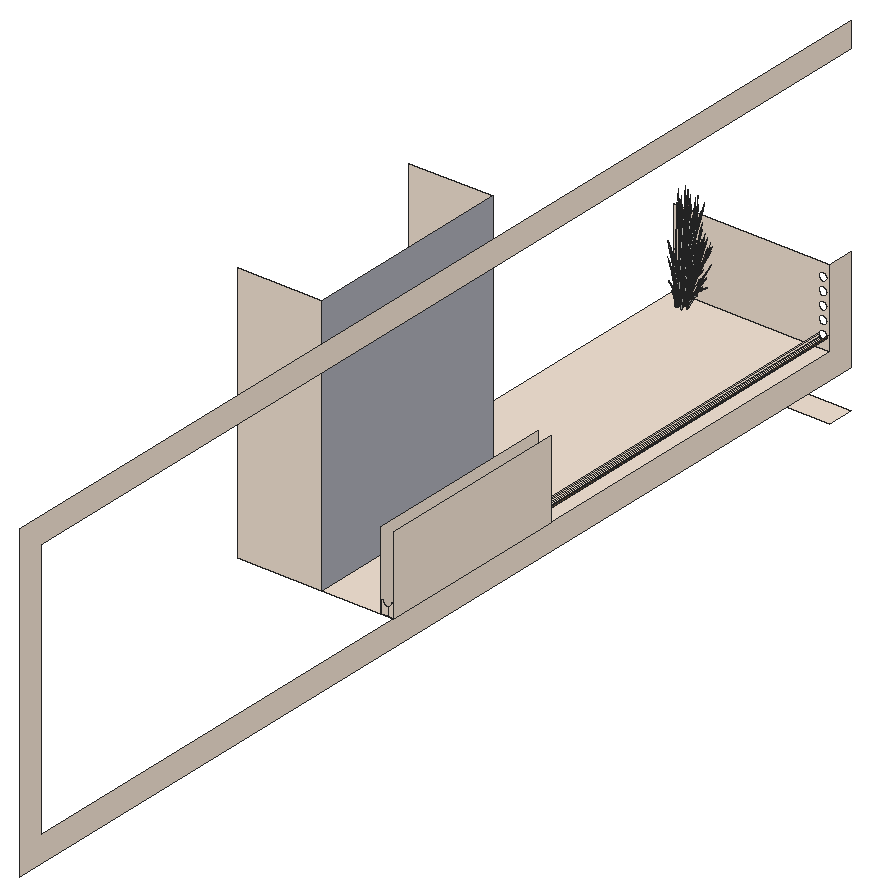
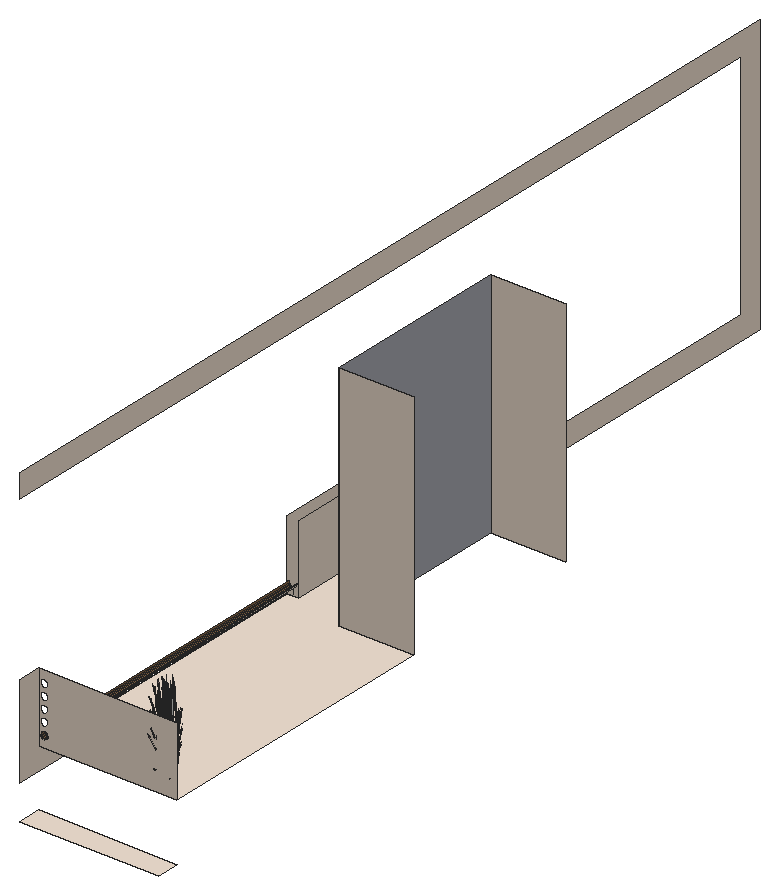
# SketchUp Ruby script. Lengths in inches.
U = 1.inch
M = Sketchup.active_model
def pt(a) = Geom::Point3d.new(a.map { |v| v * U })
def face(e, loops, mat)
  f = e.add_face(loops[0].map { |a| pt(a) })
  loops[1..].each { |l| e.add_face(l.map { |a| pt(a) }).erase! }
  f.material = f.back_material = mat if mat
  f
end
# faces: each face lists its corners as indices into pts; further lists are holes
def faces(e, pts, list, mat = nil) = list.each { |f| face(e, (f[0].is_a?(Array) ? f : [f]).map { |l| l.map { |i| pts[i] } }, mat) }
# xy, xz, yz: faces in a plane at the given z, y or x. An outline is a flat list of corners, or four numbers for a rectangle; further outlines are holes
def ring(l) = l.size == 4 ? [[l[0], l[1]], [l[2], l[1]], [l[2], l[3]], [l[0], l[3]]] : l.each_slice(2).to_a
def flat(e, list, mat, &to3) = list.each { |f| face(e, (f[0].is_a?(Array) ? f : [f]).map { |l| ring(l).map { |u, v| to3.(u, v) } }, mat) }
def xy(e, z, list, mat = nil) = flat(e, list, mat) { |x, y| [x, y, z] }
def xz(e, y, list, mat = nil) = flat(e, list, mat) { |x, z| [x, y, z] }
def yz(e, x, list, mat = nil) = flat(e, list, mat) { |y, z| [x, y, z] }
def lines(e, pts, list) = list.each { |a, b| e.add_line(pt(pts[a]), pt(pts[b])) }
# prism: a flat outline (further loops are holes) pulled along v
def prism(e, loops, v, mat = nil)
  f = face(e, loops, mat); d = Geom::Vector3d.new(v.map { |x| x * U })
  f.pushpull(f.normal.samedirection?(d) ? d.length : -d.length)
end
def box(e, o, s, mat = nil) = prism(e, [[o, [o[0] + s[0], o[1], o[2]], [o[0] + s[0], o[1] + s[1], o[2]], [o[0], o[1] + s[1], o[2]]]], [0, 0, s[2]], mat)
def at(x, y, z, deg = 0) = Geom::Transformation.translation(pt([x, y, z])) * Geom::Transformation.rotation(ORIGIN, Z_AXIS, deg.degrees)
def axes(o, x, y, z) = Geom::Transformation.new([*x, 0, *y, 0, *z, 0, *pt(o).to_a, 1])
def part(name) = M.definitions.add(name)
# library, detail: a bought-in or finely detailed component or shape, given as its bounding box
def library(name, o, s) = part(name).tap { |d| box(d.entities, o, s) }
def detail(e, o, s) = box(e.add_group.entities, o, s)
def put(e, d, t, mat = nil) = e.add_instance(d, t).tap { |i| i.material = mat if mat }
def group(e, t, mat = nil) = e.add_group.tap { |g| g.transformation = t; g.material = mat if mat }.entities
root = M.entities
M.materials.add("C01_Vanilla_Cream").color = [244, 228, 212]
M.materials.add("LightPink_Translucent").color = [144, 107, 117]
M.materials["LightPink_Translucent"].alpha = 0.75
M.materials.add("Marble_20_1K").color = [172, 173, 182]
M.materials.add("Wood_Floor_01_1K").color = [146, 111, 76]
c1 = part("blade")
p = [[2.15,0.21,22],[0,0.17,0],[0.09,0.45,0],[2.18,0.31,22],[2.29,0.31,22],[0.38,0.45,0],
  [2.48,0.24,33],[2.49,0.24,33],[2.48,0.22,33]]
faces(c1.entities,p,[[0,1,2,3],[4,5,2,3],[6,3,4,7],[8,0,3,6]])
c2 = part("seeds")
p = [[0.3,-0.1,1.38],[-0.01,-0.03,1.59],[-0.01,-0.03,0.03],[0.14,-0.07,-0.07],[0.29,-0.03,3],[0.15,0.01,3.11]]
faces(c2.entities,p,[[0,1,2,3],[1,0,4,5]],"LightPink_Translucent")
c3 = part("blade with seeds")
put(c3.entities,c1,at(0,0,0))
put(c3.entities,c2,axes([2.4,0.25,30.99],[1.5799,-0.05474,1.17369],[-0.12525,1.92788,0.29478],[-0.07173,-0.02425,1.56792]))
xy(root,132,[[288,468,360,480]],"C01_Vanilla_Cream")
xy(root,162,[[326.85,216,354,216,354,306.76,360,306.76,360,468,288,468,288,314.71,326.85,314.71],[354,216,360,306.76]],"C01_Vanilla_Cream")
xz(root,216,[[288,162,326.85,282],[354,162,357,162,357,166,356.48,166.07,356,166.27,355.59,166.59,355.27,167,355.07,167.48,355,168,354,168],[357,162,360,162,360,168,359,168,358.93,167.48,358.73,167,358.41,166.59,358,166.27,357.52,166.07,357,166]],"C01_Vanilla_Cream")
xz(root,306.76,[[354,162,354,168,355,168,355.07,167.48,355.27,167,355.59,166.59,356,166.27,356.48,166.07,357,166,357,162],[357,162,357,166,357.52,166.07,358,166.27,358.41,166.59,358.73,167,358.93,167.48,359,168,360,168,360,162]],"C01_Vanilla_Cream")
xz(root,314.71,[[288,162,326.85,282]],"C01_Vanilla_Cream")
xz(root,468,[[[288,162,360,198],[357,190,356.48,190.07,356,190.27,355.59,190.59,355.27,191,355.07,191.48,355,192,355.07,192.52,355.27,193,355.59,193.41,356,193.73,356.48,193.93,357,194,357.52,193.93,358,193.73,358.41,193.41,358.73,193,358.93,192.52,359,192,358.93,191.48,358.73,191,358.41,190.59,358,190.27,357.52,190.07],[357,184,356.48,184.07,356,184.27,355.59,184.59,355.27,185,355.07,185.48,355,186,355.07,186.52,355.27,187,355.59,187.41,356,187.73,356.48,187.93,357,188,357.52,187.93,358,187.73,358.41,187.41,358.73,187,358.93,186.52,359,186,358.93,185.48,358.73,185,358.41,184.59,358,184.27,357.52,184.07],[357,178,356.48,178.07,356,178.27,355.59,178.59,355.27,179,355.07,179.48,355,180,355.07,180.52,355.27,181,355.59,181.41,356,181.73,356.48,181.93,357,182,357.52,181.93,358,181.73,358.41,181.41,358.73,181,358.93,180.52,359,180,358.93,179.48,358.73,179,358.41,178.59,358,178.27,357.52,178.07],[357,172,356.48,172.07,356,172.27,355.59,172.59,355.27,173,355.07,173.48,355,174,355.07,174.52,355.27,175,355.59,175.41,356,175.73,356.48,175.93,357,176,357.52,175.93,358,175.73,358.41,175.41,358.73,175,358.93,174.52,359,174,358.93,173.48,358.73,173,358.41,172.59,358,172.27,357.52,172.07],[357,166,356.48,166.07,356,166.27,355.59,166.59,355.27,167,355.07,167.48,355,168,355.07,168.52,355.27,169,355.59,169.41,356,169.73,356.48,169.93,357,170,357.52,169.93,358,169.73,358.41,169.41,358.73,169,358.93,168.52,359,168,358.93,167.48,358.73,167,358.41,166.59,358,166.27,357.52,166.07]]],"C01_Vanilla_Cream")
yz(root,326.85,[[216,162,314.71,282]],"Marble_20_1K")
yz(root,354,[[216,162,306.76,198]],"C01_Vanilla_Cream")
yz(root,360,[[0,150,480,150,480,198,468,198,468,162,12,162,12,282,480,282,480,294,0,294],[216,162,306.76,198]],"C01_Vanilla_Cream")
p = [[357,306.76,166],[356.48,306.76,166.07],[356.48,468,166.07],[357,468,166],[357.52,306.76,166.07],[357.52,468,166.07],
  [356,306.76,166.27],[356,468,166.27],[358,306.76,166.27],[358,468,166.27],[355.59,306.76,166.59],[355.59,468,166.59],
  [358.41,306.76,166.59],[358.41,468,166.59],[355.27,306.76,167],[355.27,468,167],[358.73,306.76,167],[358.73,468,167],
  [355.07,306.76,167.48],[355.07,468,167.48],[358.93,306.76,167.48],[358.93,468,167.48],[355,306.76,168],[355,468,168],
  [359,306.76,168],[359,468,168]]
faces(root,p,[[0,1,2,3],[1,6,7,2],[6,10,11,7],[10,14,15,11],[14,18,19,15],[18,22,23,19]],"C01_Vanilla_Cream")
faces(root,p,[[4,0,3,5],[8,4,5,9],[12,8,9,13],[16,12,13,17],[20,16,17,21],[24,20,21,25]],"Wood_Floor_01_1K")
put(root,c3,axes([297.36,461.41,163.12],[0.0901,-0.02681,1.32257],[0.54199,0.14755,-0.20205],[0.01585,0.1663,0.22528]))
put(root,c3,axes([297.48,461.5625,165.39],[-0.16784,0.37886,-0.2656],[-0.48968,-0.1105,0.3429],[0.0449,0.15254,0.65611]))
put(root,c3,axes([298.75,459.68,163.66],[-0.27012,0.44393,-0.33554],[-0.56127,-0.21365,0.16149],[0,0.10233,1.07733]))
put(root,c3,axes([298.47,457.17,165.55],[0.41024,-0.16744,0.04823],[0.2008,0.30532,0.37966],[-0.03962,-0.13459,0.57892]))
put(root,c3,axes([297.13,462.23,165.54],[0.07057,0.07933,1.31208],[0.56952,0.03117,-0.2075],[0.05727,0.17496,0.10523]))
put(root,c3,axes([299.82,459.41,163.86],[-0.43742,-0.35886,0.13232],[0.44081,-0.34807,0.26315],[-0.04831,0.07329,1.20305]))
put(root,c3,axes([298.3125,459.2,163.65],[0,-0.57005,0],[0.69617,0,0],[0,0,1.34592]))
put(root,c3,axes([298.32,457.2,165.55],[0.54859,0.1288,0.36002],[-0.18759,0.42344,0.29685],[-0.03297,-0.16652,0.74497]))
put(root,c3,axes([297.66,459.31,163.82],[0.6273,0.23878,0.18048],[-0.3019,0.49615,0.37502],[0,-0.11437,1.20407]))
put(root,c3,axes([298.66,459.43,163.72],[0,0.56976,-0.04228],[-0.69617,0,0],[0,0.01791,1.34526]))
put(root,c3,axes([297.46,458.97,164.04],[-0.60457,0.03041,0.33554],[-0.05467,-0.50484,-0.16149],[0.10823,-0.05117,1.07733]))
put(root,c3,axes([297.43,461.16,165.79],[0.16784,-0.37886,0.2656],[0.48968,0.1105,-0.3429],[0.0449,0.15254,0.65611]))
put(root,c3,axes([297.18,458.11,163.86],[-0.16083,0.48962,0.13232],[-0.58854,-0.13856,0.26315],[0.10167,-0.00238,1.20305]))
put(root,c3,axes([298.33,460.53,163.72],[0.24206,0.56598,-0.04509],[-0.69162,0.19832,0],[0.00845,0.01976,1.2913]))
put(root,c3,axes([296.89,457.5,163.78],[-0.34808,-0.49367,0],[0.58235,-0.27531,-0.38706],[0.13264,-0.0627,1.22783]))
put(root,c3,axes([297.53,461.22,165.74],[0.26572,0.40059,-0.53284],[-0.54698,0.22325,0.0643],[0.06214,0.19355,0.75375]))
put(root,c3,axes([300.33,459.79,163.65],[-0.69582,-0.00394,-0.03732],[0,-0.55062,0.37457],[-0.02187,0.12535,1.18764]))
put(root,c3,axes([298.96,458.13,163.86],[-0.59825,0.13076,0.13232],[-0.14773,-0.48663,0.26315],[0.05336,0.0709,1.20305]))
put(root,c3,axes([298.35,456.31,164.07],[0.07142,0.28728,0.86145],[-0.3962,-0.15911,0.63294],[0.04263,-0.1471,0.18974]))
put(root,c3,axes([298.09,462.52,166.23],[0.38473,-0.28263,-0.04866],[0.35252,0.30954,-0.22062],[0.02482,0.08771,0.72768]))
put(root,c3,axes([297.98,458.84,163.77],[-0.46162,0.4471,0.34316],[-0.54842,-0.39467,0.13466],[0.11129,-0.04462,1.19142]))
put(root,c3,axes([298.77,459.55,163.66],[0.38863,0.31822,0],[-0.38863,0.31822,0],[0,0,1.2695]))
put(root,c3,axes([298.77,459.18,164.04],[0.27012,-0.44393,0.33554],[0.56127,0.21365,-0.16149],[0,0.10233,1.07733]))
put(root,c3,axes([298.53,460.72,163.65],[0.56127,0.22118,0],[-0.27012,0.45959,0],[0,0,1.31215]))
put(root,c3,axes([297.73,461.3,165.51],[0.54728,0.1235,-0.38324],[-0.18759,0.42344,-0.29685],[0.05018,0.17048,0.7333]))
put(root,c3,axes([297.26,461.32,165.78],[0.54481,-0.22937,-0.0912],[0.26773,0.4071,-0.50621],[0.07188,0.17155,0.76918]))
put(root,c3,axes([298.58,459.07,163.79],[-0.70367,-0.1038,0.36899],[0.1432,-0.58624,0.1448],[0.10283,0.05661,1.2811]))
put(root,c3,axes([300.05,456.78,165.53],[-0.05654,0.03763,1.33037],[-0.55396,-0.12696,-0.12571],[-0.02005,-0.16422,0.23543]))
put(root,c3,axes([299.61,457.86,165.78],[-0.61188,-0.02441,-0.0912],[0.01672,-0.46217,-0.50621],[0.0425,-0.178,0.76918]))
put(root,c3,axes([300.18,459.87,163.52],[-0.38863,0.30738,-0.23233],[-0.38863,-0.30738,0.23233],[0,0.09901,1.0423]))
put(root,c3,axes([299.07,459.8125,163.57],[0.20414,0.45107,-0.51909],[-0.58805,0.16245,-0.13624],[0.02256,0.15274,1.1458]))
put(root,c3,axes([298.78,459.33,163.65],[0.62289,0,0],[0,0.51004,0],[0,0,1.33805]))
put(root,c3,axes([299.37,457.94,165.79],[-0.3767,0.25939,0.2656],[-0.3566,-0.29618,-0.3429],[0.05426,-0.15048,0.65611]))
put(root,c3,axes([298.19,458.77,164.04],[-0.33445,-0.41351,0.33554],[0.50659,-0.29119,-0.16149],[0.10823,0.05117,1.07733]))
put(root,c3,axes([297.58,458.87,164],[-0.06488,-0.56215,-0.21822],[0.6757,-0.03399,-0.37502],[0.11898,-0.07488,1.19781]))
put(root,c3,axes([299,459.28,163.96],[0.51872,-0.14368,0.1086],[0.18165,0.41027,-0.3101],[0,0.09029,0.95058]))
put(root,c3,axes([299.19,457.69,165.51],[-0.39855,-0.33102,-0.38324],[0.42102,-0.2899,-0.29685],[0.06064,-0.16819,0.7333]))
put(root,c3,axes([298.82,459.31,164],[0.62699,0.23507,-0.21822],[-0.3019,0.49615,-0.37502],[0.0197,0.12182,1.19781]))
put(root,c3,axes([297.49,457.62,163.52],[0.51941,0.1219,-0.23233],[-0.13078,0.42928,0.23233],[0.10471,-0.0495,1.0423]))
put(root,c3,axes([298.93,457.1,163.94],[-0.15825,0.09972,1.07251],[-0.47395,-0.17454,-0.23066],[0.08785,-0.21706,0.45856]))
put(root,c3,axes([300.18,459.42,163.86],[0,-0.49266,0.37238],[0.62289,0,0],[0,0.11221,1.18128]))
put(root,c3,axes([300.45,459.88,163.51],[0,0.49266,-0.37238],[-0.62289,0,0],[0,0.11221,1.18128]))
put(root,c3,axes([298.79,461.37,165.55],[-0.55374,0.11306,0.36002],[-0.0961,-0.44351,0.29685],[0.13023,0.13071,0.74497]))
put(root,c3,axes([297.37,457.43,163.51],[0.52105,-0.24633,-0.37238],[0.31144,0.44171,0],[0.11867,-0.0561,1.18128]))
put(root,c3,axes([298.68,461.46,165.55],[-0.25304,0.31296,0.04823],[-0.36033,-0.18221,0.37966],[0.11649,0.10034,0.57892]))
put(root,c3,axes([298.04,460.43,164.91],[-0.12726,-0.15818,1.28532],[0.58807,-0.13317,0.10393],[0.13291,0.24832,0.54946]))
put(root,c3,axes([298.41,458.65,163.96],[0.1074,-0.43968,0.1086],[0.52474,0.07632,-0.3101],[0.0955,0.04515,0.95058]))
put(root,c3,axes([299.16,457.88,163.86],[-0.52105,-0.24633,0.37238],[0.31144,-0.44171,0],[0.11867,0.0561,1.18128]))
put(root,c3,axes([299.32,457.84,165.74],[0.01449,-0.45571,-0.53284],[0.61002,0.03061,0.0643],[0.06438,-0.19306,0.75375]))
put(root,c3,axes([298.7,460.46,163.64],[0.5845,-0.16716,-0.14398],[0.20539,0.48152,0.00006],[0.06452,-0.01848,1.30423]))
put(root,c3,axes([298.6,461.1,165.79],[-0.08599,-0.39682,0.2656],[0.49155,-0.10478,-0.3429],[0.13203,0.11372,0.65611]))
put(root,c3,axes([298.71,459.03,163.66],[0.33445,0.41351,-0.33554],[-0.50659,0.29119,0.16149],[0.10823,0.05117,1.07733]))
put(root,c3,axes([298.93,458.82,165.36],[-0.48108,-0.25598,1.03712],[0.50798,-0.39855,0.44749],[0.15521,0.24018,1.00248]))
put(root,c3,axes([299.57,457.57,165.39],[0.3767,-0.25939,-0.2656],[0.3566,0.29618,0.3429],[0.05426,-0.15048,0.65611]))
put(root,c3,axes([298.125,461.66,165.53],[0.00165,-0.05965,1.33037],[0.47711,-0.26315,-0.12571],[0.16572,0.09393,0.23543]))
put(root,c3,axes([299.71,457.7,165.55],[0.45752,0.02296,0.04823],[-0.01254,0.34663,0.37966],[0.04787,-0.13278,0.57892]))
put(root,c3,axes([299.66,460.9,164.07],[-0.31347,-0.14166,0.86145],[0.40476,-0.14393,0.63294],[0.10917,0.12192,0.18974]))
put(root,c3,axes([298.54,460.75,163.94],[0.00982,-0.16331,1.07251],[0.4695,-0.18242,-0.23066],[0.14493,0.19547,0.45856]))
put(root,c3,axes([300.17,457.13,165.54],[-0.00537,-0.09805,1.31208],[-0.45391,-0.28338,-0.2075],[0.07018,-0.17178,0.10523]))
put(root,c3,axes([297.98,458.4375,163.54],[0.375,-0.3703,-0.46765],[0.46584,0.33578,-0.12274],[0.15027,-0.09237,1.03225]))
put(root,c3,axes([299.57,457.67,165.55],[0.39645,0.33614,0.36002],[-0.42102,0.2899,0.29685],[0.07313,-0.15771,0.74497]))
put(root,c3,axes([299.63,458.11,163.52],[0.13078,0.42928,-0.23233],[-0.51941,0.1219,0.23233],[0.10471,0.0495,1.0423]))
put(root,c3,axes([300.61,459.51,163.78],[0.69617,0,0],[0,0.55062,-0.38706],[0,0.12541,1.22783]))
put(root,c3,axes([298.36,458.79,164],[0.56211,-0.32708,-0.21822],[0.3738,0.46216,-0.37502],[0.13869,0.04694,1.19781]))
put(root,c3,axes([299.71,461.55,164],[-0.35702,-0.01545,0.78795],[0.23577,-0.32816,0.43504],[0.14104,0.11659,0.61808]))
put(root,c3,axes([300.03,458.74,165.79],[-0.48462,0.07041,0.2656],[-0.12797,-0.4025,-0.3429],[0.13888,-0.10811,0.65611]))
put(root,c3,axes([298.63,457.61,164.91],[-0.10366,0.16934,1.28532],[-0.43488,-0.35044,0.10393],[0.19618,-0.21841,0.54946]))
put(root,c3,axes([298.56,461.31,165.78],[0.33176,-0.4217,-0.0912],[0.48044,0.24295,-0.50621],[0.16701,0.11914,0.76918]))
put(root,c3,axes([296.9375,458.5,163.2],[-0.548,0.19724,0.96696],[-0.17442,-0.56594,0.37572],[0.3365,0.00941,1.09981]))
put(root,c3,axes([300.28,458.77,165.78],[-0.515,-0.27165,-0.0912],[0.2967,-0.3934,-0.50621],[0.1455,-0.13675,0.76918]))
put(root,c3,axes([298.95,461.1,165.51],[0.54938,-0.11711,-0.38324],[0.0961,0.44351,-0.29685],[0.14756,0.1271,0.7333]))
put(root,c3,axes([299.46,457.625,163.78],[0.34808,-0.49367,0],[0.58235,0.27531,-0.38706],[0.13264,0.0627,1.22783]))
put(root,c3,axes([300.04,457.41,163.12],[-0.08333,-0.03881,1.32257],[-0.21404,-0.4336,-0.20205],[0.14439,-0.11767,0.22528]))
put(root,c3,axes([299.58,460.56,165.79],[-0.31678,-0.30846,0.2656],[0.36171,-0.29199,-0.3429],[0.18378,0.04443,0.65611]))
put(root,c3,axes([299.77,457.92,163.51],[0.52105,0.24633,-0.37238],[-0.31144,0.44171,0],[0.11867,0.0561,1.18128]))
put(root,c3,axes([299.87,460.84,165.55],[-0.02803,0.37463,0.04823],[-0.42332,-0.01027,0.37966],[0.16216,0.0392,0.57892]))
put(root,c3,axes([299.75,461.43,163.12],[0.04056,-0.07113,1.32257],[0.51066,-0.20948,-0.20205],[0.15482,0.10842,0.22528]))
put(root,c3,axes([299.91,460.73,165.55],[-0.41051,0.32462,0.36002],[-0.35404,-0.34474,0.29685],[0.1926,0.05988,0.74497]))
put(root,c3,axes([300.02,458.45,165.51],[-0.14302,-0.44985,-0.38324],[0.54163,-0.07869,-0.29685],[0.15522,-0.12083,0.7333]))
put(root,c3,axes([300.97,460.77,164.95],[-0.10656,-0.41414,-0.02619],[0.50364,-0.09521,-0.11874],[0.10517,0.02626,0.39164]))
put(root,c3,axes([300.1,459.7,165.79],[-0.46269,-0.13744,0.2656],[0.13495,-0.40096,-0.3429],[0.18628,-0.03677,0.65611]))
put(root,c3,axes([299.01,458.87,163.54],[0.57914,0.08077,-0.46765],[-0.12221,0.49823,-0.12274],[0.17283,0.06037,1.03225]))
put(root,c3,axes([301.48,459.16,163.7],[-0.34516,-0.31503,-0.04866],[0.37803,-0.28865,-0.22062],[0.10711,-0.02032,0.72768]))
put(root,c3,axes([300.6875,457.56,164.07],[-0.18544,0.25079,0.86145],[-0.15939,-0.33694,0.63294],[0.15316,-0.08443,0.18974]))
put(root,c3,axes([300.47,458.67,165.55],[0.3822,0.20719,0.04823],[-0.22252,0.29505,0.37966],[0.12254,-0.09539,0.57892]))
put(root,c3,axes([300.36,458.59,165.55],[0.13808,0.45342,0.36002],[-0.54163,0.07869,0.29685],[0.15963,-0.10664,0.74497]))
put(root,c3,axes([298.89,459.94,164.91],[-0.2068,-0.08488,1.28532],[0.42797,-0.35609,0.10393],[0.26673,0.16064,0.54946]))
put(root,c3,axes([301.55,458.66,165.53],[-0.07272,-0.00374,1.33037],[-0.30197,-0.40092,-0.12571],[0.12127,-0.13182,0.23543]))
put(root,c3,axes([300.42,458.5,165.39],[0.48462,-0.07041,-0.2656],[0.12797,0.4025,0.3429],[0.13888,-0.10811,0.65611]))
put(root,c3,axes([300.04,458.63,165.74],[0.29081,-0.38873,-0.53284],[0.5096,0.27626,0.0643],[0.17364,-0.14084,0.75375]))
put(root,c3,axes([300.52,459.82,165.55],[0.20448,0.33592,0.04823],[-0.37288,0.16442,0.37966],[0.16437,-0.03244,0.57892]))
put(root,c3,axes([300.03,460.73,165.39],[0.31678,0.30846,-0.2656],[-0.36171,0.29199,0.3429],[0.18378,0.04443,0.65611]))
put(root,c3,axes([299.67,460.76,165.78],[0.02981,-0.50103,-0.0912],[0.56442,0.01369,-0.50621],[0.21738,0.0348,0.76918]))
put(root,c3,axes([300.3,459.83,165.78],[-0.28012,-0.44611,-0.0912],[0.49717,-0.21923,-0.50621],[0.20951,-0.05886,0.76918]))
put(root,c3,axes([300.48,459.71,165.55],[-0.15729,0.44921,0.36002],[-0.51712,-0.15361,0.29685],[0.20336,-0.027,0.74497]))
put(root,c3,axes([300.16,460.46,165.54],[0.11943,-0.00833,1.31208],[0.32759,-0.38275,-0.2075],[0.21244,0.05052,0.10523]))
put(root,c3,axes([300.27,459.45,165.51],[0.15083,-0.44814,-0.38324],[0.51712,0.15361,-0.29685],[0.2082,-0.04109,0.7333]))
put(root,c3,axes([301.57,459.74,164.07],[-0.34399,0.08133,0.86145],[0.16192,-0.33614,0.63294],[0.18249,0.023,0.18974]))
put(root,c3,axes([300.46,458.28,163.94],[-0.19889,-0.01459,1.07251],[-0.20376,-0.39145,-0.23066],[0.24434,-0.11074,0.45856]))
put(root,c3,axes([300.59,459.66,165.39],[0.46269,0.13744,-0.2656],[-0.13495,0.40096,0.3429],[0.18628,-0.03677,0.65611]))
put(root,c3,axes([299.7,460.52,165.74],[0.55654,0.01186,-0.53284],[-0.03738,0.49951,0.0643],[0.23578,0.05271,0.75375]))
put(root,c3,axes([300.83,459.58,163.49],[-0.35858,0.05912,1.06187],[-0.05708,-0.47061,0.06078],[0.25115,-0.07123,0.60425]))
put(root,c3,axes([301.22,459.27,163.12],[-0.0291,-0.0748,1.32257],[0.20181,-0.43752,-0.20205],[0.20357,-0.00629,0.22528]))
put(root,c3,axes([301.41,461.16,165.53],[-0.05034,-0.04313,1.33037],[0.11012,-0.46232,-0.12571],[0.1983,-0.02954,0.23543]))
put(root,c3,axes([299.33,459.16,164.91],[-0.23093,0.01116,1.28532],[0.15319,-0.4836,0.10393],[0.32909,0.02991,0.54946]))
put(root,c3,axes([300.18,459.61,165.74],[0.48922,-0.21758,-0.53284],[0.27264,0.44789,0.0643],[0.23638,-0.05088,0.75375]))
put(root,c3,axes([301.82,459.14,165.54],[0.07726,-0.07504,1.31208],[-0.09888,-0.46032,-0.2075],[0.19384,-0.08728,0.10523]))
put(root,c3,axes([300.93,460.28,163.94],[-0.13408,-0.12117,1.07251],[0.17446,-0.40083,-0.23066],[0.27128,0.0543,0.45856]))
